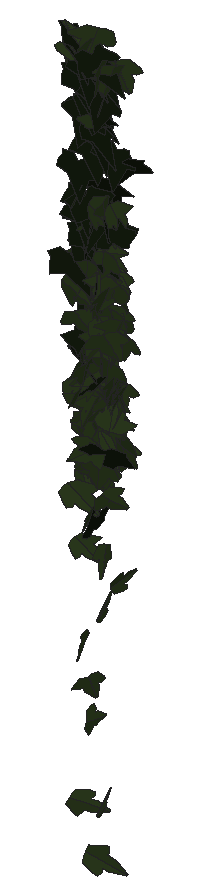
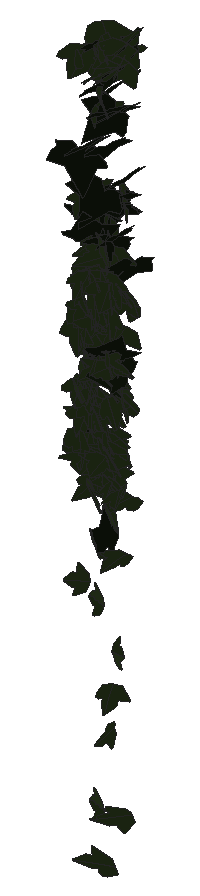
# SketchUp Ruby script. Lengths in inches.
U = 1.inch
M = Sketchup.active_model
def pt(a) = Geom::Point3d.new(a.map { |v| v * U })
def face(e, loops, mat)
  f = e.add_face(loops[0].map { |a| pt(a) })
  loops[1..].each { |l| e.add_face(l.map { |a| pt(a) }).erase! }
  f.material = f.back_material = mat if mat
  f
end
# faces: each face lists its corners as indices into pts; further lists are holes
def faces(e, pts, list, mat = nil) = list.each { |f| face(e, (f[0].is_a?(Array) ? f : [f]).map { |l| l.map { |i| pts[i] } }, mat) }
# xy, xz, yz: faces in a plane at the given z, y or x. An outline is a flat list of corners, or four numbers for a rectangle; further outlines are holes
def ring(l) = l.size == 4 ? [[l[0], l[1]], [l[2], l[1]], [l[2], l[3]], [l[0], l[3]]] : l.each_slice(2).to_a
def flat(e, list, mat, &to3) = list.each { |f| face(e, (f[0].is_a?(Array) ? f : [f]).map { |l| ring(l).map { |u, v| to3.(u, v) } }, mat) }
def xy(e, z, list, mat = nil) = flat(e, list, mat) { |x, y| [x, y, z] }
def xz(e, y, list, mat = nil) = flat(e, list, mat) { |x, z| [x, y, z] }
def yz(e, x, list, mat = nil) = flat(e, list, mat) { |y, z| [x, y, z] }
def lines(e, pts, list) = list.each { |a, b| e.add_line(pt(pts[a]), pt(pts[b])) }
# prism: a flat outline (further loops are holes) pulled along v
def prism(e, loops, v, mat = nil)
  f = face(e, loops, mat); d = Geom::Vector3d.new(v.map { |x| x * U })
  f.pushpull(f.normal.samedirection?(d) ? d.length : -d.length)
end
def box(e, o, s, mat = nil) = prism(e, [[o, [o[0] + s[0], o[1], o[2]], [o[0] + s[0], o[1] + s[1], o[2]], [o[0], o[1] + s[1], o[2]]]], [0, 0, s[2]], mat)
def at(x, y, z, deg = 0) = Geom::Transformation.translation(pt([x, y, z])) * Geom::Transformation.rotation(ORIGIN, Z_AXIS, deg.degrees)
def axes(o, x, y, z) = Geom::Transformation.new([*x, 0, *y, 0, *z, 0, *pt(o).to_a, 1])
def part(name) = M.definitions.add(name)
# library, detail: a bought-in or finely detailed component or shape, given as its bounding box
def library(name, o, s) = part(name).tap { |d| box(d.entities, o, s) }
def detail(e, o, s) = box(e.add_group.entities, o, s)
def put(e, d, t, mat = nil) = e.add_instance(d, t).tap { |i| i.material = mat if mat }
def group(e, t, mat = nil) = e.add_group.tap { |g| g.transformation = t; g.material = mat if mat }.entities
root = M.entities
M.materials.add("1026 AP 7946 SUNNY SIDE UP").color = [254, 231, 186]
M.materials.add("efeu1").color = [18, 25, 13]
M.materials.add("efeu2").color = [43, 57, 29]
c1 = part("ivyleaf_10")
p = [[0,0.5,-0.03],[-0.0625,2.02,-0.43],[-0.19,2.01,-0.46],[-0.54,1.05,-0.29],[-0.52,0.625,-0.18],[-0.83,0.76,-0.28],
  [-1.16,0.64,-0.33],[-1.15,0.33,-0.24],[-0.77,-0.39,0.02],[-0.3,-0.51,0.16],[0.04,-0.48,0.23],[-0.02,2.01,-0.4375],
  [-0.06,2.01,-0.43],[0.04,-0.49,0.23],[0.67,-0.49,0.14],[1.38,0.36,-0.2],[1.375,0.51,-0.24],[0.81,0.65,-0.19],
  [0.62,0.59,-0.15],[0.6,1.09,-0.28],[0.5,1.23,-0.31]]
faces(c1.entities,p,[[0,1,2,3,4,5,6,7,8,9,10],[11,12,0,13,14,15,16,17,18,19,20]],"efeu2")
c2 = part("ivyleaf_9")
p = [[1.54,2.16,1.25],[1.36,2.04,1.19],[-0.21,0.99,0.68],[-0.71,1.11,0.82],[-0.85,0.86,0.67],[-0.8,0.17,0.21],
  [-0.9,-0.01,0.1],[-0.67,-0.16,-0.02],[-0.08,-0.08,-0.05],[-0.03,-0.6,-0.4],[0.65,-0.88,-0.66],[0.83,-0.6,-0.49],
  [1.29,-0.42,-0.43],[1.8125,-0.07,-0.26],[1.21,0.44,0.15]]
faces(c2.entities,p,[[0,1,2,3,4,5,6,7,8,9,10,11,12,13,14]],"efeu1")
put(root,c1,axes([107.375,212.9375,258.8],[0.05135,0.2035,-0.0366],[-0.00112,-0.03703,-0.21248],[-0.32514,0.03227,-0.00505]),"1026 AP 7946 SUNNY SIDE UP")
put(root,c2,axes([107.3125,212.61,263.25],[-0.01346,-0.20228,-0.15592],[-0.00639,0.15038,-0.20752],[0.39612,-0.00445,-0.00864]),"1026 AP 7946 SUNNY SIDE UP")
put(root,c1,axes([107.51,212.67,267.43],[0.18159,0.22589,0.05465],[-0.08193,-0.03104,0.25914],[0.35507,-0.12269,0.03185]),"1026 AP 7946 SUNNY SIDE UP")
put(root,c2,axes([107.33,212.83,265.02],[-0.02031,-0.24095,0.04358],[-0.00978,-0.0434,-0.24881],[0.38493,-0.01381,-0.00402]),"1026 AP 7946 SUNNY SIDE UP")
put(root,c1,axes([107.37,212.88,262.64],[-0.32956,-0.00724,-0.09758],[0.14443,-0.07356,-0.20413],[-0.03782,-0.2179,0.07073]),"1026 AP 7946 SUNNY SIDE UP")
put(root,c1,axes([107.375,212.82,261.94],[-0.28154,-0.0954,-0.10646],[0.15339,0.03505,-0.20835],[0.15844,-0.20346,0.01253]),"1026 AP 7946 SUNNY SIDE UP")
put(root,c1,axes([107.21,212.75,262.53],[-0.08381,0.00487,-0.24827],[0.28298,-0.16343,-0.04536],[-0.25221,-0.18499,0.03161]),"1026 AP 7946 SUNNY SIDE UP")
put(root,c1,axes([107.49,212.95,259.9],[-0.08052,-0.20657,0.0306],[0.0013,-0.03199,-0.21927],[0.32842,-0.05052,0.00837]),"1026 AP 7946 SUNNY SIDE UP")
put(root,c2,axes([107.28,212.76,267.71],[0.15043,-0.24639,0.00124],[-0.00979,-0.00521,-0.27221],[0.38733,0.09556,-0.00737]),"1026 AP 7946 SUNNY SIDE UP")
put(root,c2,axes([107.23,212.9,261.16],[0.18879,-0.19676,0.09816],[0.0617,-0.08884,-0.23767],[0.33896,0.12576,-0.01141]),"1026 AP 7946 SUNNY SIDE UP")
put(root,c1,axes([107.41,212.84,262.8125],[0.24638,-0.1566,0.08243],[0.06728,-0.07122,-0.2278],[0.26887,0.16132,-0.01854]),"1026 AP 7946 SUNNY SIDE UP")
put(root,c1,axes([107.34,213.125,259.42],[0.30842,-0.14581,-0.05607],[0.08716,-0.01496,0.25081],[-0.2282,-0.20279,0.02001]),"1026 AP 7946 SUNNY SIDE UP")
put(root,c1,axes([107.52,212.88,259.11],[-0.11511,-0.19685,0.04603],[-0.01798,-0.04459,-0.21657],[0.31728,-0.07394,0.00442]),"1026 AP 7946 SUNNY SIDE UP")
put(root,c1,axes([107.49,212.65,264.6],[0.12267,-0.22434,-0.04722],[0.00295,0.04771,-0.24377],[0.35963,0.07613,0.01811]),"1026 AP 7946 SUNNY SIDE UP")
put(root,c1,axes([107.4375,212.78,267.31],[-0.14351,0.23299,-0.04692],[0.01748,-0.04596,-0.25797],[-0.37329,-0.09173,0.00595]),"1026 AP 7946 SUNNY SIDE UP")
put(root,c1,axes([107.53,212.58,260.5625],[0.0693,-0.2085,-0.08271],[-0.02245,0.07783,-0.21907],[0.34993,0.04629,0.00233]),"1026 AP 7946 SUNNY SIDE UP")
put(root,c1,axes([107.53,212.95,260.5],[-0.08903,-0.21015,0.02302],[0.00475,-0.02517,-0.22416],[0.33248,-0.05592,0.00937]),"1026 AP 7946 SUNNY SIDE UP")
put(root,c1,axes([107.375,212.85,267.59],[-0.26414,-0.12269,-0.16138],[0.2348,0.0564,-0.21108],[0.20547,-0.22217,0.03375]),"1026 AP 7946 SUNNY SIDE UP")
put(root,c1,axes([107.26,213.01,259.62],[-0.03482,-0.01713,-0.21411],[0.32571,-0.02512,-0.02076],[-0.03658,-0.2074,0.01896]),"1026 AP 7946 SUNNY SIDE UP")
put(root,c1,axes([107.34,212.89,267.27],[-0.29303,-0.05289,-0.17496],[0.2753,-0.01355,-0.19399],[0.04678,-0.25156,0.0457]),"1026 AP 7946 SUNNY SIDE UP")
put(root,c1,axes([107.75,212.88,261.33],[0.13554,-0.02465,-0.21338],[-0.31319,0.05631,-0.09203],[0.09665,0.21703,0.00101]),"1026 AP 7946 SUNNY SIDE UP")
put(root,c1,axes([107.41,212.99,259.83],[-0.26899,-0.00966,-0.12573],[0.19041,-0.04353,-0.17165],[-0.02768,-0.20555,0.041]),"1026 AP 7946 SUNNY SIDE UP")
put(root,c2,axes([107.34,212.76,267.36],[0.07545,-0.20354,0.14937],[0.05513,-0.14188,-0.21626],[0.39013,0.05942,0.00167]),"1026 AP 7946 SUNNY SIDE UP")
put(root,c2,axes([107.67,212.89,261.41],[-0.33268,-0.11154,0.08166],[0.10615,0.04322,0.24656],[-0.18782,0.22199,-0.0053]),"1026 AP 7946 SUNNY SIDE UP")
put(root,c1,axes([107.3,212.67,260.41],[0.17641,-0.07259,-0.1889],[0.26117,-0.07807,0.13638],[-0.16605,-0.19991,0.01383]),"1026 AP 7946 SUNNY SIDE UP")
put(root,c2,axes([107.42,212.76,266.89],[0.05204,-0.25829,-0.01205],[0.00102,0.01039,-0.2682],[0.40645,0.03305,0.00222]),"1026 AP 7946 SUNNY SIDE UP")
put(root,c1,axes([107.54,212.9375,258.92],[-0.01459,0.20918,-0.01736],[-0.00008,-0.01806,-0.21581],[-0.33014,-0.00924,0.00082]),"1026 AP 7946 SUNNY SIDE UP")
put(root,c1,axes([107.57,212.89,262.28],[0.27654,-0.14241,-0.05519],[0.00603,0.08487,-0.22231],[0.23872,0.16282,0.06955]),"1026 AP 7946 SUNNY SIDE UP")
put(root,c1,axes([107.65,212.87,262.93],[0.32345,-0.0713,-0.09679],[-0.10979,0.07765,-0.21868],[0.14885,0.21222,0.04904]),"1026 AP 7946 SUNNY SIDE UP")
put(root,c1,axes([107.47,212.73,257.41],[0.12153,0.15136,0.12726],[0.09429,0.10708,-0.17441],[-0.29147,0.09775,-0.00336]),"1026 AP 7946 SUNNY SIDE UP")
put(root,c1,axes([107.62,212.52,261.23],[0.02898,-0.18099,-0.13888],[0.0069,0.13449,-0.18604],[0.35383,0.0122,0.015]),"1026 AP 7946 SUNNY SIDE UP")
put(root,c1,axes([107.58,212.95,262.78],[-0.324,-0.09898,-0.04366],[0.08929,-0.02354,-0.23102],[0.14344,-0.20893,0.0452]),"1026 AP 7946 SUNNY SIDE UP")
put(root,c1,axes([107.54,212.77,255.48],[0.08945,-0.10974,0.17592],[0.12011,-0.15343,-0.12823],[0.2966,0.09523,-0.00113]),"1026 AP 7946 SUNNY SIDE UP")
put(root,c2,axes([107.42,212.92,267.125],[0.18882,-0.22044,0.04389],[0.00923,-0.04662,-0.25829],[0.3533,0.11903,-0.01671]),"1026 AP 7946 SUNNY SIDE UP")
put(root,c1,axes([107.62,212.84,261.48],[0.03305,-0.22526,0.00841],[0.05363,-0.0062,-0.23055],[0.35042,0.02219,0.03449]),"1026 AP 7946 SUNNY SIDE UP")
put(root,c1,axes([107.44,212.6,258.51],[0.201,0.14585,0.15096],[0.18164,0.09133,-0.19805],[-0.2685,0.17097,-0.02097]),"1026 AP 7946 SUNNY SIDE UP")
put(root,c2,axes([107.8,212.75,263],[0.05035,-0.04092,-0.25674],[-0.36311,0.09639,-0.04635],[0.15989,0.23179,-0.02442]),"1026 AP 7946 SUNNY SIDE UP")
put(root,c1,axes([107.6875,212.87,267.59],[-0.01652,-0.25763,0.02813],[-0.00043,-0.02878,-0.26579],[0.40761,-0.01047,0.00086]),"1026 AP 7946 SUNNY SIDE UP")
put(root,c1,axes([107.72,212.9,259.78],[-0.2677,-0.10995,0.05623],[-0.03916,-0.0615,-0.20567],[0.18945,-0.16808,0.03694]),"1026 AP 7946 SUNNY SIDE UP")
put(root,c1,axes([107.46,212.67,252.21],[-0.08742,-0.05652,-0.20249],[0.29277,0.0695,-0.07456],[0.13188,-0.19176,0.03129]),"1026 AP 7946 SUNNY SIDE UP")
put(root,c2,axes([107.56,212.84,267.07],[-0.02735,-0.2491,0.05779],[-0.01122,-0.05714,-0.25757],[0.40184,-0.01855,-0.00326]),"1026 AP 7946 SUNNY SIDE UP")
put(root,c1,axes([107.73,212.66,263.33],[-0.3537,-0.04921,0.03084],[-0.03794,-0.0303,-0.23607],[0.08249,-0.22493,0.02365]),"1026 AP 7946 SUNNY SIDE UP")
put(root,c2,axes([107.61,212.78,266.17],[-0.11197,-0.22339,0.09499],[-0.0169,-0.09442,-0.24145],[0.3804,-0.06995,0.01723]),"1026 AP 7946 SUNNY SIDE UP")
put(root,c1,axes([107.66,212.75,254.68],[-0.1556,-0.17623,-0.07444],[0.07161,0.05601,-0.20754],[0.29019,-0.10832,0.0113]),"1026 AP 7946 SUNNY SIDE UP")
put(root,c1,axes([107.7,212.5625,261.11],[-0.04322,-0.22038,-0.04271],[0.00845,0.03985,-0.22856],[0.35214,-0.02801,0.00024]),"1026 AP 7946 SUNNY SIDE UP")
put(root,c2,axes([107.59,212.76,264.48],[-0.08217,-0.23913,-0.01025],[0.01186,0.00714,-0.25205],[0.37607,-0.05247,0.00571]),"1026 AP 7946 SUNNY SIDE UP")
put(root,c1,axes([107.84,212.85,260.38],[0.22334,0.06208,-0.1562],[-0.25716,0.03602,-0.1421],[-0.02246,0.20488,0.07365]),"1026 AP 7946 SUNNY SIDE UP")
put(root,c1,axes([107.74,212.69,262.61],[0.12821,-0.17341,-0.1333],[-0.06185,0.12302,-0.19616],[0.3336,0.08945,0.01486]),"1026 AP 7946 SUNNY SIDE UP")
put(root,c2,axes([107.54,212.76,263.77],[0.07407,-0.23635,-0.06878],[-0.01714,0.06454,-0.24789],[0.38523,0.04832,0.0022]),"1026 AP 7946 SUNNY SIDE UP")
put(root,c1,axes([107.82,212.78,260.97],[0.1601,0.1115,-0.16946],[-0.2347,-0.08016,-0.15104],[-0.20754,0.17666,0.04008]),"1026 AP 7946 SUNNY SIDE UP")
put(root,c1,axes([107.66,212.75,253.87],[0.00438,-0.0529,-0.21265],[0.08107,0.20016,-0.05103],[0.32463,-0.04927,0.01561]),"1026 AP 7946 SUNNY SIDE UP")
put(root,c2,axes([107.67,212.86,266.25],[-0.18537,-0.221,0.04312],[0.00457,-0.05015,-0.25696],[0.35402,-0.11507,0.0259]),"1026 AP 7946 SUNNY SIDE UP")
put(root,c2,axes([107.64,212.91,257.6875],[0.09534,0.13797,0.20968],[-0.15222,-0.17843,0.15387],[0.35431,-0.11378,0.00969]),"1026 AP 7946 SUNNY SIDE UP")
put(root,c1,axes([107.72,212.77,259.125],[-0.11705,-0.19526,-0.03635],[0.03702,0.02754,-0.21476],[0.30948,-0.07714,0.01194]),"1026 AP 7946 SUNNY SIDE UP")
put(root,c2,axes([107.65,212.75,263.45],[-0.0037,0.15331,0.20808],[-0.10073,-0.19492,0.15117],[0.38467,-0.04957,0.04159]),"1026 AP 7946 SUNNY SIDE UP")
put(root,c1,axes([107.58,213.07,259.44],[0.24098,0.11411,0.08758],[0.09307,0.06146,-0.19604],[-0.2028,0.16379,0.01411]),"1026 AP 7946 SUNNY SIDE UP")
put(root,c1,axes([107.79,212.79,267.82],[-0.29445,-0.16811,0.0712],[-0.02512,-0.08495,-0.25444],[0.28527,-0.181,0.05109]),"1026 AP 7946 SUNNY SIDE UP")
put(root,c1,axes([107.52,212.94,258.9],[0.25054,-0.05482,-0.12952],[0.20757,0.01071,0.16802],[-0.05685,-0.20249,0.04268]),"1026 AP 7946 SUNNY SIDE UP")
put(root,c1,axes([107.86,212.59,259.5],[0.27492,-0.05794,-0.13615],[-0.20338,0.02798,-0.18922],[0.09954,0.21718,-0.01057]),"1026 AP 7946 SUNNY SIDE UP")
put(root,c1,axes([107.75,212.75,260.35],[-0.06964,-0.19301,0.11194],[0.03472,-0.11519,-0.20018],[0.34739,-0.02718,0.04245]),"1026 AP 7946 SUNNY SIDE UP")
put(root,c1,axes([107.8,212.96,260.26],[0.23723,-0.12453,-0.09324],[-0.08734,0.07309,-0.20015],[0.22506,0.15963,0.0206]),"1026 AP 7946 SUNNY SIDE UP")
put(root,c1,axes([107.77,212.84,263.63],[0.04856,-0.23499,-0.02315],[0.00003,0.02132,-0.24403],[0.371,0.03076,0.00305]),"1026 AP 7946 SUNNY SIDE UP")
put(root,c2,axes([107.6,212.78,266.23],[0.4072,-0.00034,-0.04417],[-0.06719,-0.02366,-0.26583],[-0.00555,0.26142,-0.02257]),"1026 AP 7946 SUNNY SIDE UP")
put(root,c1,axes([107.81,212.87,261.64],[-0.13372,-0.18029,0.1059],[-0.01046,-0.10974,-0.20258],[0.32696,-0.07725,0.03683]),"1026 AP 7946 SUNNY SIDE UP")
put(root,c1,axes([107.8,212.66,258.24],[0.11928,-0.21214,0.03445],[0.00858,-0.03483,-0.2322],[0.33788,0.07577,-0.00627]),"1026 AP 7946 SUNNY SIDE UP")
put(root,c2,axes([107.7,212.96,264.71],[0.37776,0.08087,-0.06339],[-0.08118,-0.04027,-0.26048],[-0.13814,0.24482,-0.02028]),"1026 AP 7946 SUNNY SIDE UP")
put(root,c2,axes([107.69,212.85,265.55],[-0.06607,-0.24416,-0.01647],[0.00535,0.01423,-0.25515],[0.38457,-0.04214,0.00072]),"1026 AP 7946 SUNNY SIDE UP")
put(root,c2,axes([107.71,212.73,264.27],[-0.15168,-0.20337,-0.09422],[0.07885,0.07603,-0.23112],[0.3409,-0.10807,0.01153]),"1026 AP 7946 SUNNY SIDE UP")
put(root,c1,axes([107.84,212.89,260.12],[-0.02003,-0.21175,0.005],[0.00491,-0.00626,-0.21855],[0.33306,-0.01264,0.00352]),"1026 AP 7946 SUNNY SIDE UP")
put(root,c2,axes([107.77,212.7,264.27],[-0.21564,-0.20073,-0.06486],[0.06317,0.0474,-0.25009],[0.32417,-0.14277,0.00559]),"1026 AP 7946 SUNNY SIDE UP")
put(root,c1,axes([107.86,212.72,263.98],[-0.07289,-0.21888,0.09284],[0.00413,-0.09356,-0.23008],[0.37292,-0.04174,0.02069]),"1026 AP 7946 SUNNY SIDE UP")
put(root,c2,axes([107.64,212.96,267.12],[0.10532,-0.23875,-0.03843],[0.01884,0.04054,-0.25419],[0.37918,0.0643,0.0233]),"1026 AP 7946 SUNNY SIDE UP")
put(root,c1,axes([107.89,212.73,266.12],[-0.09179,-0.19541,0.14922],[-0.02075,-0.14733,-0.2095],[0.38295,-0.05482,0.02442]),"1026 AP 7946 SUNNY SIDE UP")
put(root,c2,axes([107.85,212.55,260.76],[-0.18363,0.19477,-0.11223],[-0.07164,0.10083,0.23424],[0.34439,0.12483,-0.01111]),"1026 AP 7946 SUNNY SIDE UP")
put(root,c1,axes([107.66,212.9375,261.17],[0.16063,0.11747,0.16662],[0.172,0.11827,-0.15965],[-0.26206,0.14963,-0.00266]),"1026 AP 7946 SUNNY SIDE UP")
put(root,c2,axes([107.7,212.72,263.625],[0.0096,-0.18196,-0.1787],[0.05658,0.17133,-0.18394],[0.39008,-0.02037,0.03108]),"1026 AP 7946 SUNNY SIDE UP")
put(root,c1,axes([107.77,213,259.69],[-0.28574,0.03464,-0.1029],[0.14739,-0.03991,-0.1898],[-0.07751,-0.20358,0.01842]),"1026 AP 7946 SUNNY SIDE UP")
put(root,c1,axes([107.86,212.89,261.27],[-0.07422,0.2078,-0.06978],[-0.02503,-0.07357,-0.21773],[-0.34333,-0.03956,0.03096]),"1026 AP 7946 SUNNY SIDE UP")
put(root,c1,axes([107.93,212.875,262.47],[-0.02756,-0.22236,-0.07168],[0.00101,0.06846,-0.22933],[0.36576,-0.01695,-0.00477]),"1026 AP 7946 SUNNY SIDE UP")
put(root,c2,axes([107.72,212.62,264.53],[0.04277,-0.14378,-0.21673],[0.07747,0.20974,-0.14044],[0.39203,-0.02576,0.0514]),"1026 AP 7946 SUNNY SIDE UP")
put(root,c1,axes([107.93,212.75,259.03],[-0.28748,-0.11254,-0.01154],[0.02813,-0.00897,-0.22053],[0.17549,-0.18292,0.01644]),"1026 AP 7946 SUNNY SIDE UP")
put(root,c2,axes([107.77,212.86,265.72],[0.05196,-0.23715,0.07584],[0.00531,-0.07518,-0.24702],[0.39105,0.03253,-0.00672]),"1026 AP 7946 SUNNY SIDE UP")
put(root,c2,axes([108.02,212.71,263.9],[0.06658,-0.11739,0.22665],[-0.02907,0.22174,0.12647],[-0.39195,-0.03638,0.02913]),"1026 AP 7946 SUNNY SIDE UP")
put(root,c1,axes([107.88,212.77,266.41],[0.19504,-0.21046,0.0731],[0.07929,-0.05386,-0.25149],[0.34074,0.13301,0.01668]),"1026 AP 7946 SUNNY SIDE UP")
put(root,c1,axes([107.97,212.96,260.55],[-0.18882,-0.17889,0.03635],[0.01262,-0.04858,-0.21958],[0.28674,-0.11566,0.0336]),"1026 AP 7946 SUNNY SIDE UP")
put(root,c2,axes([107.97,212.97,263.73],[-0.29851,-0.06617,0.17313],[0.23515,0.08009,0.20654],[-0.16022,0.24082,-0.01944]),"1026 AP 7946 SUNNY SIDE UP")
put(root,c1,axes([107.87,212.86,261.93],[0.21549,0.1536,0.09673],[0.02327,0.10696,-0.20378],[-0.28139,0.12647,0.05722]),"1026 AP 7946 SUNNY SIDE UP")
put(root,c1,axes([108.02,212.61,259.14],[-0.32317,-0.03838,0.03377],[-0.0449,-0.026,-0.21455],[0.06572,-0.20653,0.01947]),"1026 AP 7946 SUNNY SIDE UP")
put(root,c1,axes([107.98,212.93,260.31],[-0.15596,-0.19206,-0.00237],[0.03164,-0.00904,-0.22158],[0.30033,-0.09878,0.02211]),"1026 AP 7946 SUNNY SIDE UP")
put(root,c2,axes([107.79,212.73,265.98],[0.10187,-0.24473,-0.0289],[0.01414,0.02991,-0.26009],[0.38683,0.06335,0.01712]),"1026 AP 7946 SUNNY SIDE UP")
put(root,c1,axes([107.76,212.8,263.32],[0.13113,0.09101,0.20633],[0.19982,0.15423,-0.12614],[-0.28146,0.1519,0.00658]),"1026 AP 7946 SUNNY SIDE UP")
put(root,c1,axes([108.05,212.8,262.85],[-0.22468,-0.1585,0.09324],[-0.02099,-0.10664,-0.21262],[0.28693,-0.13191,0.05746]),"1026 AP 7946 SUNNY SIDE UP")
put(root,c1,axes([108,212.8,260.53],[-0.14412,0.18994,0.05663],[-0.06258,0.04042,-0.21626],[-0.30408,-0.09835,0.01767]),"1026 AP 7946 SUNNY SIDE UP")
put(root,c1,axes([107.99,212.87,262.88],[0.31653,0.09806,-0.06361],[-0.08676,-0.029,-0.23084],[-0.16077,0.20872,-0.00068]),"1026 AP 7946 SUNNY SIDE UP")
put(root,c1,axes([108,212.9,258.63],[0.18979,-0.17294,0.00761],[-0.00881,-0.01409,-0.21696],[0.27211,0.12017,-0.01233]),"1026 AP 7946 SUNNY SIDE UP")
put(root,c1,axes([108.08,212.69,263.44],[-0.3231,0.09819,0.04964],[-0.10578,-0.03401,-0.22696],[-0.13512,-0.20817,0.05898]),"1026 AP 7946 SUNNY SIDE UP")
put(root,c1,axes([108,212.65,252.1875],[0.13092,-0.14141,0.14068],[-0.07668,0.1297,0.16877],[-0.30035,-0.09475,0.01823]),"1026 AP 7946 SUNNY SIDE UP")
put(root,c1,axes([108.24,212.84,261.94],[0.08967,0.02473,0.2306],[-0.34683,0.05201,0.05231],[-0.07034,-0.22492,0.03605]),"1026 AP 7946 SUNNY SIDE UP")
put(root,c1,axes([108.05,212.9375,259.31],[0.11111,0.19363,0.05484],[-0.03752,-0.04677,0.21197],[0.31306,-0.07432,0.00594]),"1026 AP 7946 SUNNY SIDE UP")
put(root,c2,axes([107.95,212.78,266.64],[-0.08784,-0.24052,0.0781],[-0.02953,-0.07487,-0.25482],[0.3961,-0.05892,-0.00168]),"1026 AP 7946 SUNNY SIDE UP")
put(root,c1,axes([108,212.46,264.48],[-0.05364,0.20581,0.14293],[-0.04397,0.13478,-0.21408],[-0.38677,-0.04387,0.00452]),"1026 AP 7946 SUNNY SIDE UP")
put(root,c2,axes([107.87,212.62,267.46],[0.06448,-0.20373,-0.17041],[0.00556,0.16668,-0.21109],[0.41146,0.02968,0.02956]),"1026 AP 7946 SUNNY SIDE UP")
put(root,c1,axes([107.98,212.71,267.23],[0.12215,-0.21433,0.1178],[0.09181,-0.10137,-0.2347],[0.37171,0.09547,0.01926]),"1026 AP 7946 SUNNY SIDE UP")
put(root,c1,axes([108.24,212.72,262.84],[-0.26965,-0.02142,0.15955],[-0.22905,-0.06208,-0.17524],[0.0898,-0.22266,0.0321]),"1026 AP 7946 SUNNY SIDE UP")
put(root,c1,axes([108.04,212.88,262.87],[0.23366,-0.18108,-0.02611],[-0.00701,0.02774,-0.24072],[0.28719,0.148,0.01537]),"1026 AP 7946 SUNNY SIDE UP")
put(root,c1,axes([108.05,212.83,260.76],[-0.17801,0.19136,0.02969],[-0.05137,0.01275,-0.22791],[-0.29967,-0.11586,0.02143]),"1026 AP 7946 SUNNY SIDE UP")
put(root,c1,axes([108.03,212.67,264.43],[-0.0125,-0.2291,-0.10352],[0.06526,0.09665,-0.23282],[0.38708,-0.02369,0.03591]),"1026 AP 7946 SUNNY SIDE UP")
put(root,c1,axes([108.16,212.81,262.77],[-0.28179,-0.11517,0.1046],[-0.0703,-0.11113,-0.21046],[0.23168,-0.17381,0.06336]),"1026 AP 7946 SUNNY SIDE UP")
put(root,c1,axes([108.0625,212.58,256.2],[0.11489,-0.14785,0.14742],[-0.0812,0.13473,0.17037],[-0.31413,-0.08891,0.00988]),"1026 AP 7946 SUNNY SIDE UP")
put(root,c1,axes([108.07,212.91,260.69],[0.20144,-0.17793,-0.01963],[-0.00858,0.01829,-0.22567],[0.28107,0.12807,0.00718]),"1026 AP 7946 SUNNY SIDE UP")
put(root,c1,axes([108.09,212.9,262.14],[-0.29511,0.12712,-0.01426],[-0.03421,-0.05718,-0.22569],[-0.19826,-0.17935,0.06016]),"1026 AP 7946 SUNNY SIDE UP")
put(root,c1,axes([108.19,213.04,259.66],[-0.31132,0.12762,0.10274],[-0.15341,0.03033,-0.24109],[-0.2024,-0.21928,0.02471]),"1026 AP 7946 SUNNY SIDE UP")
put(root,c1,axes([107.79,212.71,251.15],[0.07779,0.04501,0.22923],[0.33367,0.07102,-0.06306],[-0.12573,0.21633,-0.02553]),"1026 AP 7946 SUNNY SIDE UP")
put(root,c1,axes([108.11,212.63,262.75],[0.03704,-0.24056,-0.0021],[-0.00773,0.00019,-0.24896],[0.37818,0.02357,-0.00488]),"1026 AP 7946 SUNNY SIDE UP")
put(root,c1,axes([107.96,212.7,263.51],[0.00622,-0.102,-0.2332],[0.19148,0.19746,-0.08854],[0.33927,-0.10957,0.05425]),"1026 AP 7946 SUNNY SIDE UP")
put(root,c1,axes([108,212.89,260.4375],[0.34004,-0.00397,0.02559],[0.03956,0.0269,-0.2209],[0.00132,0.21601,0.02927]),"1026 AP 7946 SUNNY SIDE UP")
put(root,c1,axes([108.28,212.92,262.55],[-0.10308,0.05843,0.22152],[-0.28542,0.11539,-0.08878],[-0.20233,-0.19255,0.01238]),"1026 AP 7946 SUNNY SIDE UP")
put(root,c1,axes([108,213.12,259.38],[0.24962,0.13678,0.01087],[0.02625,-0.00443,-0.2154],[-0.21401,0.15899,-0.01374]),"1026 AP 7946 SUNNY SIDE UP")
put(root,c1,axes([108.03,212.92,262.22],[-0.34094,-0.00649,-0.07554],[0.11527,-0.0386,-0.22013],[-0.00991,-0.2256,0.03848]),"1026 AP 7946 SUNNY SIDE UP")
put(root,c2,axes([108.15,212.5625,259.5625],[0.25927,0.12067,-0.14096],[-0.15967,-0.09362,-0.21062],[-0.2393,0.19322,-0.01219]),"1026 AP 7946 SUNNY SIDE UP")
put(root,c1,axes([108.03,212.95,262.86],[-0.21482,-0.17693,-0.06884],[0.15404,0.003,-0.21778],[0.25373,-0.15162,0.07393]),"1026 AP 7946 SUNNY SIDE UP")
put(root,c1,axes([108.17,212.73,267.21],[-0.15486,-0.23848,0.04972],[0.0059,-0.055,-0.26497],[0.38297,-0.09559,0.02418]),"1026 AP 7946 SUNNY SIDE UP")
put(root,c1,axes([108.15,212.93,260.65],[0.04523,-0.21795,0.01977],[-0.00778,-0.02125,-0.22647],[0.34412,0.02816,-0.00772]),"1026 AP 7946 SUNNY SIDE UP")
put(root,c1,axes([108.12,212.97,260.09],[-0.30911,0.07821,-0.01806],[0.0146,-0.02506,-0.21715],[-0.12533,-0.19581,0.01923]),"1026 AP 7946 SUNNY SIDE UP")
put(root,c1,axes([108.21,212.64,261.27],[-0.33427,0.04032,0.04846],[-0.07906,-0.01543,-0.22162],[-0.05646,-0.21713,0.02343]),"1026 AP 7946 SUNNY SIDE UP")
put(root,c1,axes([108.03,212.71,257.44],[0.24371,-0.11892,0.12152],[0.12343,-0.09143,-0.2006],[0.23351,0.17244,-0.02079]),"1026 AP 7946 SUNNY SIDE UP")
put(root,c1,axes([108.14,212.95,260.67],[-0.29294,-0.108,-0.0324],[0.0727,-0.01932,-0.21819],[0.16094,-0.18785,0.03959]),"1026 AP 7946 SUNNY SIDE UP")
put(root,c1,axes([108.22,212.87,261.53],[0.11203,-0.18653,-0.10996],[-0.05996,0.09855,-0.20512],[0.33172,0.08081,0.00006]),"1026 AP 7946 SUNNY SIDE UP")
put(root,c2,axes([108.28,212.63,263.86],[-0.36882,-0.02163,0.06097],[0.09233,0.00902,0.24269],[-0.03644,0.24177,-0.00217]),"1026 AP 7946 SUNNY SIDE UP")
put(root,c2,axes([108.23,212.93,265.28],[0.19592,0.19761,-0.10734],[-0.08167,-0.09173,-0.24116],[-0.34249,0.13492,-0.0039]),"1026 AP 7946 SUNNY SIDE UP")
put(root,c2,axes([108.1,212.96,265.46],[-0.08018,-0.23528,0.04454],[0.00088,-0.04568,-0.24806],[0.37653,-0.04999,0.01007]),"1026 AP 7946 SUNNY SIDE UP")
put(root,c1,axes([108.27,212.95,259.42],[-0.3041,0.07149,0.05367],[-0.09337,-0.01337,-0.20989],[-0.10258,-0.19974,0.03194]),"1026 AP 7946 SUNNY SIDE UP")
put(root,c1,axes([108.22,212.78,260.94],[0.02784,-0.22211,0.02786],[-0.00071,-0.02843,-0.2297],[0.35208,0.01751,-0.00267]),"1026 AP 7946 SUNNY SIDE UP")
put(root,c1,axes([108.14,212.76,260.02],[0.33195,0.07655,-0.02736],[0.02805,0.02962,0.23044],[0.12451,-0.21076,0.02103]),"1026 AP 7946 SUNNY SIDE UP")
put(root,c1,axes([108.18,212.85,261.69],[-0.07449,0.16912,-0.14582],[-0.02078,-0.14764,-0.17684],[-0.34712,-0.02746,0.04188]),"1026 AP 7946 SUNNY SIDE UP")
put(root,c1,axes([108.27,212.96,261.73],[-0.33247,0.07047,0.03683],[-0.06658,-0.01615,-0.22783],[-0.10457,-0.21377,0.02796]),"1026 AP 7946 SUNNY SIDE UP")
put(root,c1,axes([108.28,212.81,262.07],[-0.19796,-0.18534,0.0513],[-0.03198,-0.0476,-0.23089],[0.30051,-0.12716,0.00922]),"1026 AP 7946 SUNNY SIDE UP")
put(root,c1,axes([108.23,212.97,260.66],[0.10506,-0.20133,0.05268],[0.0075,-0.05341,-0.2185],[0.32699,0.06591,-0.01192]),"1026 AP 7946 SUNNY SIDE UP")
put(root,c1,axes([108.18,212.88,256.73],[0.05734,-0.09299,0.19559],[-0.01536,0.19224,0.09978],[-0.3328,-0.02489,0.02909]),"1026 AP 7946 SUNNY SIDE UP")
put(root,c1,axes([108.14,212.63,258.62],[-0.13314,-0.13133,-0.16847],[0.16732,0.12414,-0.15947],[0.28313,-0.13512,0.01502]),"1026 AP 7946 SUNNY SIDE UP")
put(root,c1,axes([108.28,212.83,260.6875],[-0.13389,0.16149,0.12484],[-0.10215,0.10156,-0.18728],[-0.29967,-0.10677,0.00806]),"1026 AP 7946 SUNNY SIDE UP")
put(root,c1,axes([108.2,212.88,267.25],[-0.30892,-0.15259,-0.07078],[0.12815,0.00381,-0.25196],[0.22918,-0.20781,0.04548]),"1026 AP 7946 SUNNY SIDE UP")
put(root,c1,axes([108.21,212.54,261.88],[-0.26359,-0.15879,-0.09221],[0.12043,0.04764,-0.23696],[0.25933,-0.18353,0.01632]),"1026 AP 7946 SUNNY SIDE UP")
put(root,c1,axes([108.21,212.76,264.37],[0.05882,0.21777,0.08737],[-0.01449,0.08595,-0.22598],[-0.36648,0.03155,0.02295]),"1026 AP 7946 SUNNY SIDE UP")
put(root,c1,axes([108.28,212.79,260.28],[0.15329,-0.19529,-0.00532],[-0.01996,-0.00181,-0.22452],[0.3065,0.09755,-0.01196]),"1026 AP 7946 SUNNY SIDE UP")
